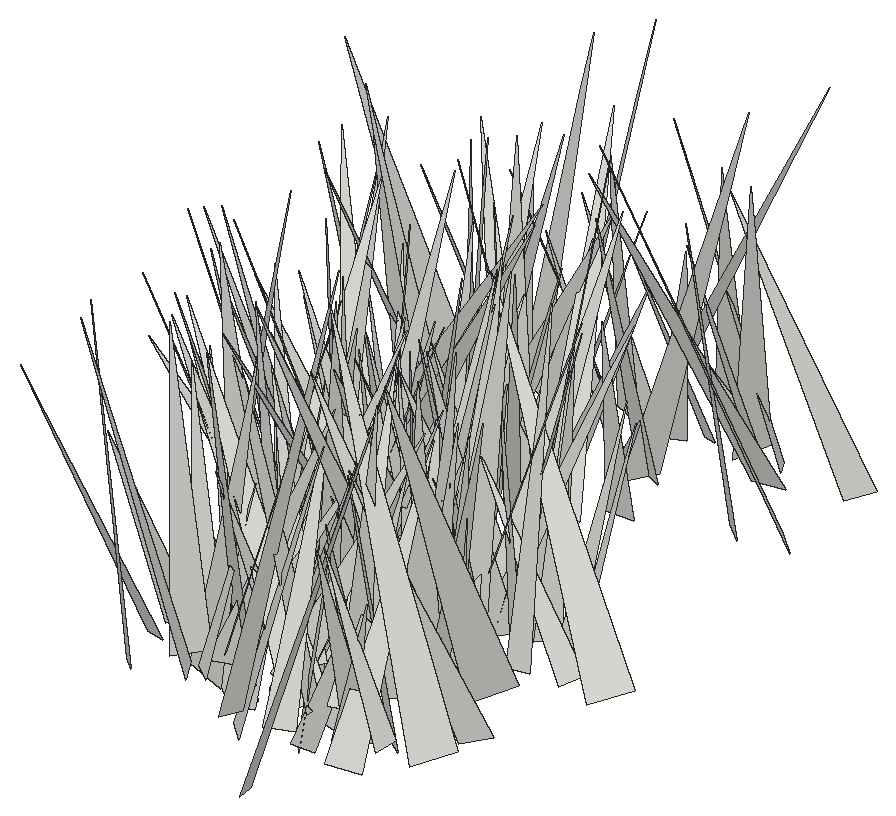
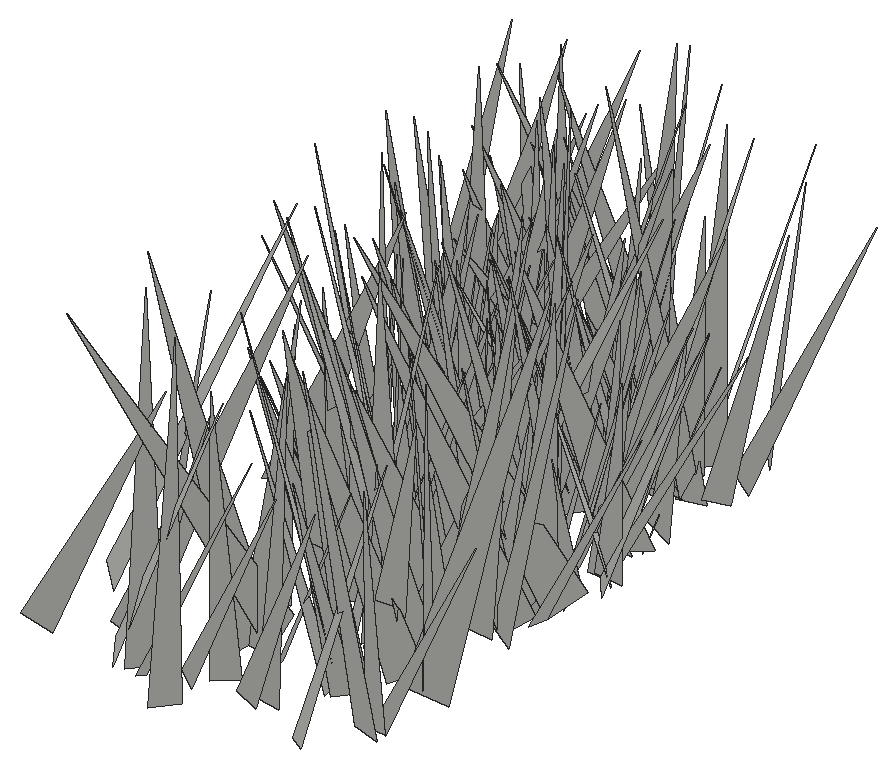
# SketchUp Ruby script. Lengths in inches.
U = 1.inch
M = Sketchup.active_model
def pt(a) = Geom::Point3d.new(a.map { |v| v * U })
def face(e, loops, mat)
  f = e.add_face(loops[0].map { |a| pt(a) })
  loops[1..].each { |l| e.add_face(l.map { |a| pt(a) }).erase! }
  f.material = f.back_material = mat if mat
  f
end
# faces: each face lists its corners as indices into pts; further lists are holes
def faces(e, pts, list, mat = nil) = list.each { |f| face(e, (f[0].is_a?(Array) ? f : [f]).map { |l| l.map { |i| pts[i] } }, mat) }
# xy, xz, yz: faces in a plane at the given z, y or x. An outline is a flat list of corners, or four numbers for a rectangle; further outlines are holes
def ring(l) = l.size == 4 ? [[l[0], l[1]], [l[2], l[1]], [l[2], l[3]], [l[0], l[3]]] : l.each_slice(2).to_a
def flat(e, list, mat, &to3) = list.each { |f| face(e, (f[0].is_a?(Array) ? f : [f]).map { |l| ring(l).map { |u, v| to3.(u, v) } }, mat) }
def xy(e, z, list, mat = nil) = flat(e, list, mat) { |x, y| [x, y, z] }
def xz(e, y, list, mat = nil) = flat(e, list, mat) { |x, z| [x, y, z] }
def yz(e, x, list, mat = nil) = flat(e, list, mat) { |y, z| [x, y, z] }
def lines(e, pts, list) = list.each { |a, b| e.add_line(pt(pts[a]), pt(pts[b])) }
# prism: a flat outline (further loops are holes) pulled along v
def prism(e, loops, v, mat = nil)
  f = face(e, loops, mat); d = Geom::Vector3d.new(v.map { |x| x * U })
  f.pushpull(f.normal.samedirection?(d) ? d.length : -d.length)
end
def box(e, o, s, mat = nil) = prism(e, [[o, [o[0] + s[0], o[1], o[2]], [o[0] + s[0], o[1] + s[1], o[2]], [o[0], o[1] + s[1], o[2]]]], [0, 0, s[2]], mat)
def at(x, y, z, deg = 0) = Geom::Transformation.translation(pt([x, y, z])) * Geom::Transformation.rotation(ORIGIN, Z_AXIS, deg.degrees)
def axes(o, x, y, z) = Geom::Transformation.new([*x, 0, *y, 0, *z, 0, *pt(o).to_a, 1])
def part(name) = M.definitions.add(name)
# library, detail: a bought-in or finely detailed component or shape, given as its bounding box
def library(name, o, s) = part(name).tap { |d| box(d.entities, o, s) }
def detail(e, o, s) = box(e.add_group.entities, o, s)
def put(e, d, t, mat = nil) = e.add_instance(d, t).tap { |i| i.material = mat if mat }
def group(e, t, mat = nil) = e.add_group.tap { |g| g.transformation = t; g.material = mat if mat }.entities
root = M.entities
c1 = part("fur_instance\#9")
p = [[0.8125,0,1.79],[0.67,-0.02,1.48],[0,-0.11,0],[0,0.11,0]]
faces(c1.entities,p,[[0,1,2,3]])
put(root,c1,axes([65.08,203.15,-27.1],[-4.61833,-3.74237,0.73758],[-3.79853,4.40694,-1.4242],[-0.34716,1.56584,5.77113]))
put(root,c1,axes([64.76,215.15,-27.1],[-2.53868,-3.44184,0.53172],[-3.38696,2.28677,-1.36858],[-0.81085,1.22404,4.05193]))
put(root,c1,axes([65.04,206.53,-27.1],[-4.32306,0.06447,0.02072],[0.06687,4.27292,0.65655],[0.01068,-0.65679,4.2734]))
put(root,c1,axes([64.88,212.69,-27.1],[1.74253,-7.39949,2.19817],[-7.33714,-2.28781,-1.88496],[-2.39807,1.62304,7.36449]))
put(root,c1,axes([65.42,202.29,-27.1],[-4.70731,-0.314,0.0439],[-0.28456,4.4722,1.47573],[0.13983,-1.46975,4.48103]))
put(root,c1,axes([66.14,203.4,-27.1],[-6.00367,-1.40851,0.07652],[-1.40991,5.98159,-0.51624],[-0.04369,0.52005,6.14503]))
put(root,c1,axes([65.65,195,-27.1],[-2.53227,-4.93937,0.36335],[-4.86121,2.40071,-1.24381],[-0.94765,0.88376,5.4095]))
put(root,c1,axes([65.08,202.77,-27.1],[-0.91318,4.58049,0.90258],[4.61205,0.74242,0.89849],[-0.72428,-1.04754,4.5834]))
put(root,c1,axes([65.41,208.03,-27.1],[-3.32824,-5.52708,1.61735],[-5.74671,3.30884,-0.51825],[0.37393,1.65668,6.43096]))
put(root,c1,axes([66.1875,192.95,-27.1],[-4.69579,-3.74143,2.09942],[-4.25802,4.44495,-1.60248],[0.52452,2.58851,5.78625]))
put(root,c1,axes([64.71,215.53,-27.1],[-0.60793,-4.00143,1.69165],[-4.28266,0.83877,0.44495],[0.72934,1.58988,4.02282]))
put(root,c1,axes([67.04,199.72,-27.1],[-3.88022,2.75048,0.41463],[2.75578,3.70465,1.21426],[-0.37781,-1.22622,4.59857]))
put(root,c1,axes([65.375,202.37,-27.1],[4.3588,4.87451,1.02077],[4.50794,-4.43827,1.9448],[-2.11691,0.58556,6.24322]))
put(root,c1,axes([67.14,204.19,-28.22],[-5.44191,5.3364,0.6963],[5.36336,5.45938,0.07682],[0.44311,-0.54257,7.6214]))
put(root,c1,axes([66.73,202.41,-27.1],[-6.28754,-2.52373,1.27093],[-2.51372,6.41179,0.29625],[1.29062,0.19325,6.76865]))
put(root,c1,axes([65.23,212.08,-27.1],[-4.85936,-1.80324,2.4582],[-1.94231,5.39639,0.11902],[2.34986,0.73149,5.18178]))
put(root,c1,axes([65.54,196.49,-27.1],[3.46395,-3.11936,0.86631],[-2.7787,-3.51575,-1.54862],[-1.66124,-0.62369,4.39672]))
put(root,c1,axes([67.02,197.71,-28.22],[0.45308,4.94253,1.25959],[4.74966,-0.86975,1.70432],[-1.859,-1.01755,4.66145]))
put(root,c1,axes([66.02,203.7,-27.1],[1.84085,7.01016,1.12106],[6.97031,-2.00445,1.08846],[-1.34679,-0.79226,7.16563]))
put(root,c1,axes([66.19,200.5,-27.1],[-4.76858,-5.56642,0.65425],[-5.40433,4.79429,1.40014],[1.48534,-0.42682,7.19472]))
put(root,c1,axes([64.84,215.89,-27.1],[2.76981,6.05425,2.08045],[6.39697,-2.70498,-0.64491],[-0.24704,-2.16406,6.62646]))
put(root,c1,axes([66.65,198.87,-28.22],[-3.14416,-1.79317,0.28571],[-1.75542,3.14785,0.43854],[0.46429,-0.24163,3.59289]))
put(root,c1,axes([66.24,217.81,-27.1],[-3.01664,-4.03882,0.35129],[-3.9528,3.02747,0.86334],[0.90049,-0.2406,4.96657]))
put(root,c1,axes([66.43,203.5,-28.22],[-3.11694,-3.18155,0.61605],[-3.14817,3.17551,0.47138],[0.76862,0.10457,4.42892]))
put(root,c1,axes([66.89,208.97,-27.1],[6.73753,-0.02978,4.19134],[0.53715,-7.86314,-0.91932],[-4.15689,-1.06433,6.67458]))
put(root,c1,axes([65.95,210.21,-27.1],[0.08928,4.21713,1.27448],[4.4055,-0.088,-0.01741],[-0.00879,-1.27457,4.21804]))
put(root,c1,axes([67.82,211.23,-27.1],[-2.82943,5.24506,0.49337],[5.22615,2.72388,1.01368],[-0.66438,-0.91081,5.87271]))
put(root,c1,axes([68.02,193.8,-27.1],[-5.59539,-3.44886,0.89561],[-3.54081,5.56848,-0.67808],[0.39927,1.05,6.53783]))
put(root,c1,axes([67.28,205.88,-27.1],[0.68239,3.8164,1.4602],[3.78451,-1.14857,1.23331],[-1.54098,-1.13076,3.67553]))
put(root,c1,axes([68.09,208.93,-27.1],[-3.16334,-6.14078,0.476],[-6.132,3.08971,-0.89149],[-0.57823,0.82883,6.8499]))
put(root,c1,axes([66.33,208.27,-27.1],[-0.95753,-7.17721,1.84222],[-7.39469,1.0444,0.22542],[0.47406,1.79439,7.23729]))
put(root,c1,axes([66.2,210.7,-27.1],[3.99026,4.07334,2.14881],[4.32029,-4.29562,0.12027],[-1.59518,-1.44473,5.70086]))
put(root,c1,axes([67.6,202.66,-28.22],[-2.9488,-2.48385,0.84804],[-2.61567,2.88641,-0.64107],[0.2167,1.04076,3.80183]))
put(root,c1,axes([67.57,200.3125,-27.1],[-2.05359,-3.75931,0.63579],[-3.81243,2.01617,-0.39286],[-0.04503,0.74602,4.26559]))
put(root,c1,axes([69.12,198.18,-28.22],[-3.27496,5.22829,1.96451],[5.47571,2.5569,2.32348],[-1.10043,-2.83671,5.71505]))
put(root,c1,axes([66.96,199.28,-28.22],[-3.2389,7.2108,0.31573],[7.08918,3.2432,-1.34571],[1.35602,0.26802,7.78942]))
put(root,c1,axes([67.55,195.52,-27.1],[1.73924,-4.25815,2.51532],[-4.74882,-2.1825,-0.41111],[-1.38108,2.14207,4.58125]))
put(root,c1,axes([66.69,201.22,-28.22],[-0.80762,-5.18,0.70533],[-5.16495,0.90095,0.70267],[0.80822,0.5814,5.19528]))
put(root,c1,axes([67.32,194.8,-27.1],[-4.56803,3.68378,2.77525],[4.20348,4.93276,0.37129],[1.89817,-2.05836,5.85656]))
put(root,c1,axes([68.58,203.9,-27.1],[-4.8792,2.06982,0.10093],[1.96371,4.70056,-1.46614],[0.66196,1.31208,5.09325]))
put(root,c1,axes([65.96,206.77,-27.1],[1.53162,3.70831,1.75315],[4.01532,-0.97314,-1.44953],[0.83802,-2.1148,3.74116]))
put(root,c1,axes([67.2,205.1,-27.1],[-4.37143,-2.8181,2.86453],[-3.24687,4.97094,-0.06453],[2.3675,1.61389,5.20067]))
put(root,c1,axes([66.41,210.89,-27.1],[6.19902,-0.22924,1.58295],[-0.50577,-6.29178,1.06951],[-1.51739,1.16065,6.11037]))
put(root,c1,axes([67.49,199.83,-27.1],[2.92591,-1.89098,1.19539],[-1.88086,-3.14489,-0.37117],[-1.21125,0.31559,3.46396]))
put(root,c1,axes([67.06,196.01,-27.1],[7.33246,2.99097,2.42144],[2.72494,-7.71469,1.27771],[-2.71735,0.33456,7.81527]))
put(root,c1,axes([68.26,203.83,-28.22],[-2.19445,-3.56039,1.55722],[-3.85398,2.22319,-0.34801],[0.4981,1.5159,4.16783]))
put(root,c1,axes([71.12,201.22,-28.22],[-5.59942,-5.49473,0.70955],[-5.42162,5.22657,-2.3104],[-1.14084,2.13071,7.49717]))
put(root,c1,axes([68.85,207.0625,-27.1],[-5.84983,3.65343,0.11485],[3.32744,5.4123,-2.68634],[1.51292,2.22277,6.35229]))
put(root,c1,axes([66.65,202.92,-27.1],[3.46775,1.51161,0.84573],[1.722,-3.21287,-1.3182],[-0.18693,-1.55498,3.54578]))
put(root,c1,axes([67.02,214.33,-27.1],[2.18192,-3.03993,1.35648],[-3.32882,-1.9865,0.90262],[0.01238,1.6293,3.63142]))
put(root,c1,axes([69.35,216.57,-27.1],[-0.15517,3.72025,1.9318],[3.94772,-0.52047,1.31942],[-1.40985,-1.86683,3.48188]))
put(root,c1,axes([68.74,203.81,-28.22],[-3.51503,-1.89548,0.64915],[-1.82323,3.56963,0.55065],[0.83071,-0.18586,3.95538]))
put(root,c1,axes([68.97,198.53,-28.22],[-6.10704,-5.17922,1.29191],[-4.99805,6.23748,1.37932],[1.87424,-0.24245,7.88782]))
put(root,c1,axes([68.9,210.33,-27.1],[-3.88558,0.60859,0.85055],[0.43871,3.91906,-0.80001],[0.9494,0.67978,3.85072]))
put(root,c1,axes([67.8,203.21,-27.1],[1.8777,6.7714,0.98346],[6.8334,-1.90815,0.09124],[-0.35155,-0.923,7.02632]))
put(root,c1,axes([68.25,197.23,-27.1],[2.83404,-7.21043,2.36501],[-7.48804,-3.06648,-0.37599],[-1.22999,2.05469,7.73827]))
put(root,c1,axes([65.43,207.12,-27.1],[6.30652,-2.10429,0.15189],[-2.07978,-6.12031,1.56194],[0.35446,1.52876,6.46224]))
put(root,c1,axes([69.98,200.78,-28.22],[-3.1759,-6.57357,0.78945],[-6.61199,3.10387,-0.75436],[-0.34161,1.03711,7.26148]))
put(root,c1,axes([64.98,205.04,-27.1],[6.90826,-2.9112,0.5406],[-2.88435,-6.30625,2.89882],[0.66922,2.87186,6.91346]))
put(root,c1,axes([69.95,214.11,-27.1],[-3.92921,-1.09616,0.24918],[-1.11465,3.91653,-0.34741],[0.14562,0.40197,4.06442]))
put(root,c1,axes([68.23,210.68,-27.1],[-4.38219,4.14776,3.28171],[4.71988,4.98997,-0.0042],[2.38668,-2.25242,6.03386]))
put(root,c1,axes([67.97,213.39,-27.1],[5.71474,5.0925,1.62445],[5.00095,-5.93344,1.00766],[-1.88756,-0.30227,7.58791]))
put(root,c1,axes([69.17,197.35,-27.1],[1.62899,5.48386,2.82302],[6.01922,-2.05055,0.50999],[-1.34582,-2.53344,5.69792]))
put(root,c1,axes([69.25,211.16,-27.1],[-4.71687,-4.84842,1.35584],[-4.8132,4.8877,0.73342],[1.47602,0.44449,6.72444]))
put(root,c1,axes([67.17,213.54,-27.1],[1.41484,-4.55258,1.06253],[-4.54528,-1.07998,1.42506],[1.09333,1.40157,4.54939]))
put(root,c1,axes([66.6,204.5,-28.22],[-1.50636,-7.45489,0.25307],[-6.77182,1.47502,3.14252],[3.12761,-0.39686,6.92598]))
put(root,c1,axes([67.15,199.49,-28.22],[2.30365,5.6713,0.71156],[5.64313,-2.13475,-1.25489],[0.90837,-1.12069,5.9913]))
put(root,c1,axes([66.17,212.07,-27.1],[4.35594,-4.3452,0.48537],[-4.22774,-4.01128,2.03138],[1.11472,1.7662,5.80763]))
put(root,c1,axes([67.42,195.43,-28.22],[-0.42435,-6.57592,2.54627],[-6.78158,1.0798,1.65847],[1.93298,2.34469,6.37748]))
put(root,c1,axes([69.36,196.78,-27.1],[4.53649,3.63122,1.57008],[3.09166,-4.74451,2.04009],[-2.46831,0.73111,5.44092]))
put(root,c1,axes([68.62,216.33,-27.1],[-1.39495,-5.41554,1.57218],[-5.52882,1.63221,0.71678],[1.10996,1.3242,5.54619]))
put(root,c1,axes([68.21,201.68,-28.22],[-0.43128,5.47544,2.09207],[5.72554,0.84273,-1.02531],[1.25517,-1.9628,5.39585]))
put(root,c1,axes([68.46,193.98,-27.1],[2.21445,2.95218,0.72503],[3.03203,-2.20951,-0.26401],[-0.21871,-0.73996,3.68096]))
put(root,c1,axes([69.24,200.32,-27.1],[-4.9247,-5.05159,2.9073],[-5.39927,5.38751,0.21521],[2.19519,1.91829,7.05159]))
put(root,c1,axes([69.75,194.55,-28.22],[-4.70225,1.57903,0.9136],[0.9953,4.33742,-2.37389],[1.52885,2.03289,4.35536]))
put(root,c1,axes([67.61,214.29,-27.1],[4.85217,1.44436,0.49792],[1.4914,-4.83766,-0.50049],[-0.33141,-0.62336,5.03778]))
put(root,c1,axes([67.83,196.84,-27.1],[1.33461,3.80482,0.72121],[3.71713,-1.04467,-1.36733],[1.08616,-1.09999,3.79319]))
put(root,c1,axes([71.16,197.93,-28.22],[-1.35626,4.67986,0.4324],[4.48876,1.15652,1.56235],[-1.3925,-0.82998,4.61514]))
put(root,c1,axes([67.9375,196.03,-27.1],[5.69643,3.12279,1.00252],[3.16084,-5.76326,-0.00802],[-0.87518,-0.48903,6.49623]))
put(root,c1,axes([72.51,194.48,-27.1],[-5.71185,4.45959,0.23835],[4.39877,5.55102,1.55146],[-0.77178,-1.36683,7.07857]))
put(root,c1,axes([71.02,196.5625,-27.1],[-4.64621,2.31988,0.55706],[2.32982,4.67441,-0.03457],[0.51391,-0.21773,5.19306]))
put(root,c1,axes([68.95,195.81,-28.22],[-3.46246,-6.72611,1.90114],[-6.59046,3.84836,1.61233],[2.32826,0.89059,7.39118]))
put(root,c1,axes([69.04,198.51,-28.22],[2.36922,2.94645,1.17355],[3.15581,-2.33594,-0.5062],[-0.31572,-1.23846,3.7468]))
put(root,c1,axes([69.75,203.57,-27.1],[3.22406,2.21993,1.84513],[2.48282,-3.54361,-0.0749],[-1.47248,-1.11442,3.91371]))
put(root,c1,axes([72.93,194.46,-27.1],[-7.75285,-2.01113,0.68817],[-2.11722,7.53738,-1.82488],[0.1887,1.94117,7.79879]))
put(root,c1,axes([69.31,197.85,-28.22],[2.29816,3.3477,0.63042],[3.39972,-2.30202,-0.16916],[-0.21536,-0.61617,4.05709]))
put(root,c1,axes([71.22,206.17,-27.1],[-4.01235,0.08097,0.58825],[0.14386,4.03101,0.42638],[0.5761,-0.44265,3.99045]))
put(root,c1,axes([69.51,204.16,-27.1],[5.12051,1.66894,1.66295],[1.70709,-5.37015,0.13306],[-1.62376,-0.38277,5.38398]))
put(root,c1,axes([70.8,195.71,-27.1],[0.6809,-4.24063,0.83858],[-4.19337,-0.85411,-0.91428],[-1.04966,0.66131,4.19651]))
put(root,c1,axes([69.25,199.04,-27.1],[4.51704,3.2359,0.24642],[3.07452,-4.40221,1.45028],[-1.0388,1.04161,5.3639]))
put(root,c1,axes([71.04,202.63,-27.1],[-4.89796,-0.50596,1.28828],[-0.38248,5.0478,0.52832],[1.33018,-0.4116,4.8956]))
put(root,c1,axes([71.75,216.71,-27.1],[-2.18116,-3.44946,0.52539],[-3.41914,1.9894,-1.13316],[-0.6959,1.0372,3.92074]))
put(root,c1,axes([71.08,209.45,-27.1],[-3.48559,6.14429,0.41822],[6.11379,3.5101,-0.61419],[0.74073,-0.05879,7.03735]))
put(root,c1,axes([68.62,194.96,-27.1],[4.54931,-2.96003,1.24819],[-3.21199,-4.22741,1.68171],[-0.05363,2.09362,5.16041]))
put(root,c1,axes([71.41,200.44,-28.22],[-4.60941,2.24833,0.68921],[2.12734,4.63308,-0.88638],[1.00221,0.50623,5.05134]))
put(root,c1,axes([73.32,198.25,-28.22],[0.20171,6.63601,2.13173],[6.14884,-1.17367,3.07178],[-3.28217,-1.79094,5.8857]))
put(root,c1,axes([68.05,195.4375,-28.22],[3.26284,4.45559,0.15103],[4.26787,-3.06768,-1.7017],[1.28856,-1.1217,5.25381]))
put(root,c1,axes([68.6,199.68,-27.1],[5.57249,-4.36069,0.56036],[-4.38496,-5.5781,0.19774],[-0.31889,0.50141,7.07313]))
put(root,c1,axes([69.49,205.12,-27.1],[3.75751,0.05108,0.3502],[0.07903,-3.76142,-0.29936],[-0.34497,-0.30538,3.74592]))
put(root,c1,axes([73.32,202.29,-27.1],[-3.16767,-3.69393,0.44061],[-3.42422,2.66901,-2.24153],[-1.45395,1.76199,4.31912]))
put(root,c1,axes([71.97,205.72,-27.1],[3.98122,4.30027,2.75674],[4.211,-4.74141,1.31475],[-2.89126,-0.98426,5.71085]))
put(root,c1,axes([73.86,199.25,-27.1],[-2.5504,-6.61055,0.06946],[-6.29815,2.40698,-2.17909],[-2.00934,0.84606,6.74207]))
put(root,c1,axes([71.98,204.75,-27.1],[-4.35378,0.44066,1.23045],[0.84047,4.2213,1.46212],[1.0009,-1.62788,4.12453]))
put(root,c1,axes([70.93,192.42,-27.1],[7.1916,2.06862,2.54607],[1.20326,-7.37063,2.58975],[-3.05186,1.96861,7.0208]))
put(root,c1,axes([69.93,204.02,-28.22],[7.18044,-3.7228,0.21814],[-3.29243,-6.55088,-3.42221],[-1.75122,-2.94828,7.32847]))
put(root,c1,axes([68.92,208.88,-27.1],[5.69332,3.04756,1.30745],[3.31373,-5.12843,-2.47574],[0.12746,-2.79687,5.96424]))
put(root,c1,axes([72.41,200.39,-28.22],[0.98136,-7.62341,0.77855],[-7.49654,-1.11781,-1.49599],[-1.58884,0.56543,7.53933]))
put(root,c1,axes([70.36,198.5,-28.22],[7.59105,-2.36712,2.02897],[-2.18853,-7.84946,-0.96967],[-2.22043,-0.35586,7.89221]))
put(root,c1,axes([69.82,207.09,-27.1],[0.42063,-4.67833,0.35233],[-4.37367,-0.26302,1.72907],[1.69763,0.48155,4.36738]))
put(root,c1,axes([70.56,193.17,-28.22],[3.76051,3.97563,0.83952],[4.01253,-3.81366,0.08642],[-0.64034,-0.54974,5.47171]))
put(root,c1,axes([73.61,195.4,-28.22],[2.76553,6.92914,2.18566],[6.51494,-3.40021,2.53621],[-3.21647,-0.92942,7.01632]))
put(root,c1,axes([71.57,213.62,-27.1],[-1.87294,-5.65903,1.00828],[-5.62978,2.02003,0.87988],[1.16052,0.66634,5.89562]))
put(root,c1,axes([70.7,215.97,-27.1],[2.83156,-3.99697,0.33188],[-4.00855,-2.80696,0.39506],[0.13188,0.49882,4.88236]))
put(root,c1,axes([72.9,197.14,-27.1],[-1.18349,4.29439,0.91251],[4.36217,1.04349,0.74676],[-0.49586,-1.06979,4.39144]))
put(root,c1,axes([70,210.74,-27.1],[4.56637,-2.19972,0.30987],[-2.21681,-4.46657,0.96025],[0.14341,0.99877,4.97679]))
put(root,c1,axes([70.18,195.39,-28.22],[4.49917,3.28934,0.87918],[3.40387,-4.3112,-1.28935],[0.07989,-1.55853,5.42216]))
put(root,c1,axes([72.83,192.6,-27.1],[-4.26385,3.34064,0.29483],[3.15748,4.15963,-1.468],[1.13011,0.98225,5.21395]))
put(root,c1,axes([73.08,217.47,-27.1],[-3.99864,-1.03805,0.42764],[-0.78188,3.71014,1.695],[0.80565,-1.55139,3.76744]))
put(root,c1,axes([70.78,196.06,-28.22],[3.47844,1.93474,0.04271],[1.93521,-3.47755,-0.07868],[0.00093,-0.08952,3.97952]))
put(root,c1,axes([71.78,203.12,-28.22],[-0.06431,5.36711,1.48252],[5.54585,0.19413,-0.46222],[0.49719,-1.47116,5.34755]))
put(root,c1,axes([71.29,201.4375,-28.22],[-0.94911,6.39885,1.08787],[6.32075,1.1611,-1.31509],[1.4754,-0.85797,6.33377]))
put(root,c1,axes([74.79,198.11,-28.22],[-8.06314,0.9505,0.88883],[1.02226,8.07835,0.63476],[0.80526,-0.7379,8.09412]))
put(root,c1,axes([74.77,216.76,-27.1],[-5.23852,-3.39609,0.6769],[-3.443,4.97658,-1.67721],[-0.37061,1.77027,6.01352]))
put(root,c1,axes([71.19,218.5625,-27.1],[5.82388,-2.11588,0.96568],[-1.89422,-5.82584,-1.34106],[-1.34958,-0.95373,6.04946]))
put(root,c1,axes([70.47,207.87,-27.1],[-2.5118,-6.70095,1.69222],[-6.07027,2.9998,2.86854],[3.30427,0.41708,6.55616]))
put(root,c1,axes([74.44,198.46,-27.1],[-0.7633,-7.78268,1.04828],[-7.63293,0.4877,-1.93706],[-1.84592,1.20152,7.57632]))
put(root,c1,axes([74.26,199.46,-27.1],[-4.45422,0.97791,0.2811],[1.01486,4.3608,0.91044],[0.07343,-0.95002,4.4685]))
put(root,c1,axes([72.46,199.91,-28.22],[0.90222,6.95991,0.72818],[6.98982,-0.93156,0.24337],[-0.33621,-0.69025,7.01392]))
put(root,c1,axes([73,199.91,-27.1],[-1.62337,4.08317,1.17277],[4.21606,1.70273,-0.09236],[0.52201,-1.05424,4.39307]))
put(root,c1,axes([72.91,199.6875,-27.1],[4.10406,6.33899,0.98584],[6.11766,-4.2195,1.66374],[-1.93105,0.10466,7.36601]))
put(root,c1,axes([71.18,198.42,-27.1],[2.09245,-2.98815,0.44058],[-2.87886,-1.81085,1.39087],[0.91397,1.13723,3.37237]))
put(root,c1,axes([72.71,202.26,-27.1],[-0.45657,6.34549,1.8425],[6.59681,0.54314,-0.23589],[0.37708,-1.81886,6.35752]))
put(root,c1,axes([72.83,193.61,-28.22],[3.02903,2.92229,1.12241],[2.89072,-3.2105,0.55771],[-1.2014,-0.35704,4.17178]))
put(root,c1,axes([73.32,203.58,-28.22],[3.35042,-5.0359,1.55374],[-4.92978,-3.64566,-1.18576],[-1.86322,0.59037,5.93123]))
put(root,c1,axes([73.7,194.98,-27.1],[-2.14385,5.53708,0.23418],[5.53457,2.15208,-0.21752],[0.2875,-0.13964,5.93364]))
put(root,c1,axes([72.22,197.77,-27.1],[-0.22733,-5.68785,1.31588],[-5.73337,0.46581,1.02292],[1.10075,1.2515,5.59972]))
put(root,c1,axes([71.18,212.4,-27.1],[7.74445,1.42991,0.81828],[1.0012,-7.20795,3.11989],[-1.30836,2.94814,7.231]))
put(root,c1,axes([74.5,201.52,-28.22],[-3.17,-4.98135,1.74667],[-5.27871,2.99065,-1.05117],[-0.00204,2.03858,5.81015]))
put(root,c1,axes([71.57,213.28,-27.1],[7.18053,-1.42617,1.70446],[-1.71997,-7.21687,1.20732],[-1.40743,1.54336,7.22055]))
put(root,c1,axes([73,193.63,-28.22],[-5.44791,2.04028,1.98238],[0.64646,5.0587,-3.42987],[2.77031,2.83181,4.69878]))
put(root,c1,axes([72.625,210.86,-27.1],[0.91835,-4.65892,0.5996],[-4.68613,-0.86646,0.44487],[0.32448,0.67241,4.72768]))
put(root,c1,axes([72.52,197.26,-28.22],[-0.56005,-4.94681,0.27227],[-4.82604,0.60667,1.09544],[1.12,0.14049,4.85639]))
put(root,c1,axes([73.65,204.48,-27.1],[5.66789,4.81372,1.80284],[4.22946,-5.89252,2.43659],[-2.92126,0.80836,7.02566]))
put(root,c1,axes([74.44,216.09,-27.1],[-1.9055,-4.08481,0.78377],[-4.15591,1.83492,-0.5407],[-0.16841,0.93717,4.47485]))
put(root,c1,axes([71.14,195,-27.1],[0.71966,5.69009,1.64056],[5.43341,0.02279,-2.46251],[2.35511,-1.79132,5.17987]))
put(root,c1,axes([72.86,200.35,-28.22],[5.93404,-1.49093,1.99542],[-1.59561,-6.23409,0.08712],[-1.91274,0.57506,6.11785]))
put(root,c1,axes([71.21,205.99,-27.1],[5.75664,2.23558,0.62086],[2.31995,-5.52205,-1.62697],[0.03364,-1.74108,5.95732]))
put(root,c1,axes([75.2,215.54,-27.1],[-0.88458,-7.33954,0.10795],[-7.20369,0.84713,-1.43254],[-1.40973,0.27658,7.25253]))
put(root,c1,axes([74.61,199.35,-27.1],[1.33499,-4.14938,1.03511],[-3.92508,-1.61935,-1.42916],[-1.69781,0.48101,4.1179]))
put(root,c1,axes([74.04,202.73,-28.22],[-2.39227,-3.29447,0.41561],[-3.24315,2.42809,0.57931],[0.71291,-0.00928,4.03]))
put(root,c1,axes([73.88,200.09,-27.1],[-3.9744,-0.24759,1.6573],[0.13335,4.20562,0.94807],[1.67038,-0.92483,3.8676]))
put(root,c1,axes([74.54,204.21,-28.22],[-3.84179,0.25674,0.88435],[-0.00822,3.78425,-1.13434],[0.92083,1.10494,3.67947]))
put(root,c1,axes([72.81,204.02,-28.22],[0.33819,7.69063,1.05021],[7.70297,-0.20312,-0.99305],[0.95553,-1.08446,7.63374]))
put(root,c1,axes([72.72,202.49,-27.1],[2.84119,-6.18581,2.36185],[-6.62137,-2.65127,1.02137],[0.00779,2.57322,6.73004]))
put(root,c1,axes([75.7,196.45,-28.22],[-6.21207,0.31771,0.7174],[0.09871,5.99609,-1.80072],[0.77837,1.77522,5.95384]))
put(root,c1,axes([73.34,190.15,-28.22],[6.96857,3.90701,1.2479],[3.36407,-6.85211,2.66731],[-2.34628,1.77954,7.53068]))
put(root,c1,axes([73.99,200.23,-28.22],[-3.33376,-1.76985,1.3611],[-1.54667,3.5947,0.88593],[1.61021,-0.21143,3.66899]))
put(root,c1,axes([76.27,197.64,-28.22],[-6.62778,2.24684,1.33683],[2.5489,6.36376,1.94128],[0.58185,-2.2841,6.72363]))
put(root,c1,axes([73.58,206.25,-27.1],[4.19942,-1.36084,1.21546],[-1.38514,-4.36301,-0.09922],[-1.1877,0.2767,4.41329]))
put(root,c1,axes([74.76,204.4,-28.22],[-4.76791,1.69378,1.39092],[1.4281,4.92716,-1.10462],[1.66255,0.62512,4.93778]))
put(root,c1,axes([73.46,195.8125,-27.1],[0.07384,-6.03784,2.03973],[-6.28438,0.27016,1.02718],[1.05955,2.02311,5.95028]))
put(root,c1,axes([73.47,200.47,-27.1],[0.57309,-4.07864,0.58369],[-4.03575,-0.43699,0.90892],[0.82985,0.69149,4.01716]))
put(root,c1,axes([73.33,195.15,-28.22],[0.44835,5.06558,1.88586],[5.29017,-0.02286,-1.19629],[1.10933,-1.93829,4.94267]))
put(root,c1,axes([73.39,216.92,-27.1],[5.78336,-2.78291,1.02515],[-2.6557,-5.85961,-0.92463],[-1.32013,-0.40388,6.35113]))
put(root,c1,axes([75.2,195.67,-28.22],[-2.97615,-4.05495,1.48787],[-4.26463,3.04523,-0.23114],[0.68511,1.34083,5.02461]))
put(root,c1,axes([74.28,195.1,-28.22],[2.27929,-4.31761,0.37807],[-4.29346,-2.30768,-0.46977],[-0.59235,0.11282,4.85966]))
put(root,c1,axes([75.22,202.12,-27.1],[1.82668,3.73793,1.95155],[3.99067,-2.21946,0.51574],[-1.36206,-1.48974,4.1283]))
put(root,c1,axes([73.72,199.32,-28.22],[0.25447,-5.59234,1.88155],[-5.79418,0.11887,1.13692],[1.11444,1.89496,5.48146]))
put(root,c1,axes([73.8,194.82,-28.22],[1.922,-3.18961,0.22781],[-3.1707,-1.86642,0.61867],[0.41494,0.51232,3.67219]))
put(root,c1,axes([73.19,204.01,-27.1],[3.15484,4.86518,0.39731],[4.85003,-3.07066,-0.91053],[0.55227,-0.82578,5.72659]))
put(root,c1,axes([74.16,198.55,-28.22],[5.8288,-3.89293,1.62458],[-3.86791,-6.0381,-0.59132],[-1.68328,0.3943,6.98428]))
put(root,c1,axes([72.625,204.65,-28.22],[6.83601,2.20523,1.02382],[2.40175,-6.59991,-1.82073],[-0.37792,-2.05437,6.94831]))
put(root,c1,axes([74.92,193.375,-28.22],[-2.73527,5.15415,0.70761],[4.98067,2.82527,-1.3261],[1.50298,0.0175,5.68229]))
put(root,c1,axes([78.07,194.22,-27.1],[-7.19785,3.45896,0.52945],[3.49375,7.17168,0.64382],[0.19618,-0.81015,7.95983]))
put(root,c1,axes([77.12,202.71,-28.22],[-3.7614,2.09395,0.36046],[2.10674,3.58022,1.1859],[-0.27609,-1.20834,4.13841]))
put(root,c1,axes([76.33,193.87,-27.1],[-3.68845,0.83243,0.84341],[0.99836,3.66829,0.74556],[0.6384,-0.92717,3.70698]))
put(root,c1,axes([78.1,212.84,-27.1],[-5.60021,-5.8066,0.30959],[-5.79691,5.54128,-0.92996],[-0.45638,0.8674,8.01337]))
put(root,c1,axes([76.51,200.6,-27.1],[1.43264,6.02249,0.66756],[5.77311,-1.565,1.72927],[-1.84042,-0.22107,5.94411]))
put(root,c1,axes([76.25,212.32,-27.1],[-3.7574,-4.18768,1.74578],[-4.4509,3.84178,-0.36412],[0.87968,1.55129,5.61445]))
put(root,c1,axes([78.01,216.84,-27.1],[-2.55985,4.83206,1.74885],[4.89019,1.69025,2.4878],[-1.579,-2.59892,4.86955]))
put(root,c1,axes([74.13,199.96,-28.22],[-0.76172,-5.93829,1.58025],[-5.83151,1.20063,1.7008],[1.93753,1.27903,5.74028]))
put(root,c1,axes([78.82,202.67,-28.22],[-5.54363,5.04114,0.10568],[4.92423,5.3789,1.72499],[-1.08457,-1.34553,7.29173]))
put(root,c1,axes([77.15,197.61,-28.22],[1.50286,-5.49819,1.33251],[-5.18917,-1.88889,-1.94134],[-2.25347,0.68284,5.35909]))
put(root,c1,axes([74.1875,199.27,-28.22],[6.13982,-1.63324,0.91897],[-1.58888,-6.20592,-0.4139],[-0.99371,-0.16841,6.33984]))
put(root,c1,axes([76.09,203.57,-28.22],[-4.08665,1.67614,0.95166],[1.15635,3.91687,-1.93308],[1.54207,1.50482,3.97156]))
put(root,c1,axes([75.68,200.37,-28.22],[5.79186,-5.56058,1.06137],[-5.14067,-5.80215,-2.34538],[-2.37068,-1.00358,7.67886]))
put(root,c1,axes([76.49,203.62,-28.22],[2.09645,3.63188,0.13416],[3.39461,-2.01213,1.42535],[-1.29816,0.60366,3.94386]))
